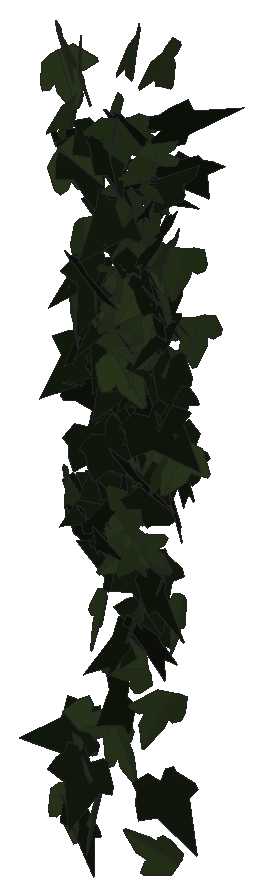
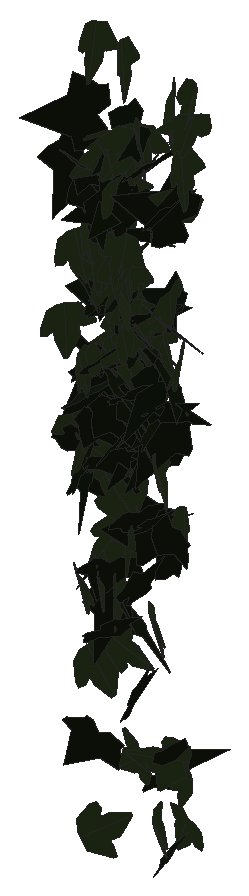
# SketchUp Ruby script. Lengths in inches.
U = 1.inch
M = Sketchup.active_model
def pt(a) = Geom::Point3d.new(a.map { |v| v * U })
def face(e, loops, mat)
  f = e.add_face(loops[0].map { |a| pt(a) })
  loops[1..].each { |l| e.add_face(l.map { |a| pt(a) }).erase! }
  f.material = f.back_material = mat if mat
  f
end
# faces: each face lists its corners as indices into pts; further lists are holes
def faces(e, pts, list, mat = nil) = list.each { |f| face(e, (f[0].is_a?(Array) ? f : [f]).map { |l| l.map { |i| pts[i] } }, mat) }
# xy, xz, yz: faces in a plane at the given z, y or x. An outline is a flat list of corners, or four numbers for a rectangle; further outlines are holes
def ring(l) = l.size == 4 ? [[l[0], l[1]], [l[2], l[1]], [l[2], l[3]], [l[0], l[3]]] : l.each_slice(2).to_a
def flat(e, list, mat, &to3) = list.each { |f| face(e, (f[0].is_a?(Array) ? f : [f]).map { |l| ring(l).map { |u, v| to3.(u, v) } }, mat) }
def xy(e, z, list, mat = nil) = flat(e, list, mat) { |x, y| [x, y, z] }
def xz(e, y, list, mat = nil) = flat(e, list, mat) { |x, z| [x, y, z] }
def yz(e, x, list, mat = nil) = flat(e, list, mat) { |y, z| [x, y, z] }
def lines(e, pts, list) = list.each { |a, b| e.add_line(pt(pts[a]), pt(pts[b])) }
# prism: a flat outline (further loops are holes) pulled along v
def prism(e, loops, v, mat = nil)
  f = face(e, loops, mat); d = Geom::Vector3d.new(v.map { |x| x * U })
  f.pushpull(f.normal.samedirection?(d) ? d.length : -d.length)
end
def box(e, o, s, mat = nil) = prism(e, [[o, [o[0] + s[0], o[1], o[2]], [o[0] + s[0], o[1] + s[1], o[2]], [o[0], o[1] + s[1], o[2]]]], [0, 0, s[2]], mat)
def at(x, y, z, deg = 0) = Geom::Transformation.translation(pt([x, y, z])) * Geom::Transformation.rotation(ORIGIN, Z_AXIS, deg.degrees)
def axes(o, x, y, z) = Geom::Transformation.new([*x, 0, *y, 0, *z, 0, *pt(o).to_a, 1])
def part(name) = M.definitions.add(name)
# library, detail: a bought-in or finely detailed component or shape, given as its bounding box
def library(name, o, s) = part(name).tap { |d| box(d.entities, o, s) }
def detail(e, o, s) = box(e.add_group.entities, o, s)
def put(e, d, t, mat = nil) = e.add_instance(d, t).tap { |i| i.material = mat if mat }
def group(e, t, mat = nil) = e.add_group.tap { |g| g.transformation = t; g.material = mat if mat }.entities
root = M.entities
M.materials.add("efeu1").color = [18, 25, 13]
M.materials.add("efeu2").color = [43, 57, 29]
c1 = part("ivyleaf_9")
p = [[1.54,2.16,1.25],[1.36,2.04,1.19],[-0.21,0.99,0.68],[-0.71,1.11,0.82],[-0.85,0.86,0.67],[-0.8,0.17,0.21],
  [-0.9,-0.01,0.1],[-0.67,-0.16,-0.02],[-0.08,-0.08,-0.05],[-0.03,-0.6,-0.4],[0.65,-0.88,-0.66],[0.83,-0.6,-0.49],
  [1.29,-0.42,-0.43],[1.8125,-0.07,-0.26],[1.21,0.44,0.15]]
faces(c1.entities,p,[[0,1,2,3,4,5,6,7,8,9,10,11,12,13,14]],"efeu1")
c2 = part("ivyleaf_10")
p = [[0,0.5,-0.03],[-0.0625,2.02,-0.43],[-0.19,2.01,-0.46],[-0.54,1.05,-0.29],[-0.52,0.625,-0.18],[-0.83,0.76,-0.28],
  [-1.16,0.64,-0.33],[-1.15,0.33,-0.24],[-0.77,-0.39,0.02],[-0.3,-0.51,0.16],[0.04,-0.48,0.23],[-0.02,2.01,-0.4375],
  [-0.06,2.01,-0.43],[0.04,-0.49,0.23],[0.67,-0.49,0.14],[1.38,0.36,-0.2],[1.375,0.51,-0.24],[0.81,0.65,-0.19],
  [0.62,0.59,-0.15],[0.6,1.09,-0.28],[0.5,1.23,-0.31]]
faces(c2.entities,p,[[0,1,2,3,4,5,6,7,8,9,10],[11,12,0,13,14,15,16,17,18,19,20]],"efeu2")
put(root,c1,axes([562.42,130.92,237.73],[0.53828,-0.80602,-0.202],[-0.09043,0.18243,-0.9689],[0.82601,0.54523,0.02556]))
put(root,c1,axes([563.375,131.01,223.55],[0.65129,-0.48232,0.57917],[0.49242,-0.30719,-0.80957],[0.5706,0.81562,0.03758]))
put(root,c1,axes([561.1875,131.4,209.32],[-0.31246,-0.89852,0.09086],[-0.02999,-0.08576,-0.9513],[0.9026,-0.3139,-0.00015]))
put(root,c1,axes([561.04,131.21,231.3],[0.42093,-0.46544,0.73818],[0.51312,-0.53091,-0.62735],[0.70587,0.66349,0.01585]))
put(root,c1,axes([561.99,131.15,238.16],[0.17865,-0.96038,-0.15125],[0.17379,0.18285,-0.95577],[0.95656,0.14614,0.20189]))
put(root,c2,axes([563.16,130.71,228.33],[0.71443,0.30335,0.61866],[0.54056,0.30587,-0.77422],[-0.42727,0.8942,0.05495]))
put(root,c2,axes([561.73,130.32,240.95],[-0.39643,0.28971,0.97126],[-0.77878,0.58041,-0.49098],[-0.64868,-0.87386,-0.00411]))
put(root,c2,axes([565.5,130.67,242.87],[-0.07993,-0.92921,-0.42172],[0.05156,0.41879,-0.93253],[1.01912,-0.09407,0.0141]))
put(root,c2,axes([564.62,130.75,236.61],[-0.9146,0.32449,0.01296],[-0.01122,0.00714,-0.97045],[-0.32456,-0.91466,-0.00298]))
put(root,c1,axes([565.01,130.58,226.54],[-0.14596,-0.31953,-0.94406],[0.31855,0.88913,-0.35019],[0.9444,-0.34929,-0.02778]))
put(root,c1,axes([564.41,130.8,232.36],[0.67031,-0.622,-0.34601],[-0.19163,0.30004,-0.91059],[0.68548,0.69211,0.08379]))
put(root,c1,axes([563.4,130.91,215.93],[-0.80632,0.58689,-0.0241],[0.01185,-0.02466,-0.99721],[-0.58727,-0.80631,0.01296]))
put(root,c2,axes([563.54,130.99,235.85],[-0.65715,0.56335,-0.47401],[0.37812,-0.28693,-0.86521],[-0.63172,-0.75776,-0.02478]))
put(root,c1,axes([565.68,131.09,231.25],[-0.96323,0.50519,-0.32722],[0.28967,-0.15219,-1.08767],[-0.52762,-1.00584,0.00022]))
put(root,c2,axes([563.14,130.9,238.87],[-0.82898,-0.58294,-0.0186],[0.01115,0.01647,-1.0134],[0.58313,-0.82902,-0.00706]))
put(root,c2,axes([565.11,131.35,213.51],[-0.37294,-0.87684,0.45217],[-0.1122,-0.44256,-0.95076],[0.98016,-0.38429,0.06321]))
put(root,c2,axes([560.35,130.8125,241.84],[-0.77246,0.62242,0.08901],[-0.0651,0.06107,-0.992],[-0.62537,-0.77517,-0.00668]))
put(root,c1,axes([560.81,131.17,220.22],[0.46178,0.1007,-0.92747],[0.91364,0.16047,0.47232],[0.18867,-1.02357,-0.0172]))
put(root,c1,axes([564.52,130.97,218.94],[0.67957,-0.63242,-0.33134],[-0.22317,0.24635,-0.92794],[0.67818,0.71478,0.02666]))
put(root,c1,axes([562.83,131.7,234.74],[-0.81509,-0.53147,0.11797],[0.04162,-0.27261,-0.94058],[0.54282,-0.77715,0.24926]))
put(root,c1,axes([563.21,130.78,239.23],[1.00852,-0.06202,-0.08568],[-0.08469,0.01875,-1.01034],[0.06338,1.01198,0.01347]))
put(root,c2,axes([563.74,131.01,242.74],[0.28145,-0.94142,-0.25988],[-0.00186,0.26994,-0.97987],[0.97663,0.27182,0.07303]))
put(root,c2,axes([562.89,131.58,232.83],[0.26327,-0.71145,0.6138],[0.45024,-0.46398,-0.73091],[0.82474,0.4804,0.20308]))
put(root,c2,axes([563.62,131.4,236.32],[-0.34525,-0.90146,0.24674],[-0.02997,-0.25222,-0.96343],[0.93414,-0.34126,0.06028]))
put(root,c2,axes([564.58,131.3,231.3],[0.94867,-0.22191,0.05992],[0.05955,-0.0085,-0.97426],[0.22201,0.95052,0.00527]))
put(root,c2,axes([563.8125,131.36,231.99],[0.8586,0.38619,-0.3853],[-0.36742,-0.1217,-0.94074],[-0.40324,0.93319,0.03677]))
put(root,c2,axes([562.69,131.36,239.25],[0.6154,-0.78959,0.04184],[0.09138,0.01836,-0.99762],[0.7854,0.61654,0.08328]))
put(root,c2,axes([564.27,131.65,228.75],[-0.36525,-0.76946,0.49291],[-0.0791,-0.50221,-0.84259],[0.91037,-0.35235,0.12455]))
put(root,c1,axes([564.98,131.26,209.82],[-0.30449,-0.36779,-0.9293],[0.73072,0.58084,-0.46931],[0.68185,-0.78672,0.08795]))
put(root,c2,axes([560.42,131.22,238.71],[0.06764,-0.98974,-0.17322],[-0.00006,0.17361,-0.99198],[1.00478,0.06664,0.01161]))
put(root,c1,axes([565.03,130.86,231.29],[0.0181,0.13265,-1.05903],[-1.0673,0.00589,-0.01751],[0.00367,1.05917,0.13273]))
put(root,c2,axes([560.14,131.03,240.64],[0.42511,0.86432,0.23318],[0.08388,0.21854,-0.96299],[-0.89128,0.43282,0.02059]))
put(root,c1,axes([562.86,131.15,229.47],[0.86,-0.39274,-0.06197],[-0.0508,0.03793,-0.94534],[0.39434,0.86139,0.01337]))
put(root,c2,axes([564.41,131.39,237.95],[0.66411,-0.72675,0.02418],[0.05594,0.01841,-0.98301],[0.72499,0.66429,0.0537]))
put(root,c2,axes([563.24,131.125,230.125],[-0.83326,-0.3656,-0.27601],[0.25782,0.09928,-0.90986],[0.37865,-0.87215,0.01213]))
put(root,c2,axes([563.79,131.36,214.59],[-0.26955,0.05015,0.89638],[-0.87007,-0.24532,-0.24792],[0.22133,-0.90331,0.11709]))
put(root,c1,axes([564.31,131.5,231.5],[0.61368,-0.6177,0.43655],[0.38239,-0.23167,-0.86535],[0.65261,0.71659,0.09654]))
put(root,c1,axes([565.86,131.27,237.02],[-0.70405,0.61197,0.32245],[-0.46019,-0.07089,-0.87026],[-0.51643,-0.77112,0.3359]))
put(root,c1,axes([564.25,130.97,216.58],[0.90189,0.14899,-0.53833],[-0.53266,-0.07835,-0.91408],[-0.16814,1.04741,0.0082]))
put(root,c2,axes([562.85,131.3,220.68],[0.57368,-0.03964,0.78885],[0.78367,0.15028,-0.56236],[-0.09861,0.96374,0.12013]))
put(root,c1,axes([562.49,132.1,212.51],[-0.07871,-0.49549,0.82496],[-0.1517,-0.81097,-0.50157],[0.95029,-0.1705,-0.01174]))
put(root,c2,axes([563.39,131.41,229.0625],[-0.74927,-0.55932,0.22375],[-0.15598,-0.16479,-0.93425],[0.58187,-0.7644,0.03769]))
put(root,c2,axes([560.67,130.82,236.61],[0.32302,0.79126,0.65933],[0.26155,0.60533,-0.85459],[-0.99619,0.4155,-0.01057]))
put(root,c1,axes([562.15,131.65,229.22],[-0.78545,-0.26057,-0.4574],[0.44405,0.11328,-0.82706],[0.28271,-0.90184,0.02827]))
put(root,c2,axes([563.29,131.78,219.8],[0.34467,0.38691,-0.74989],[-0.52499,-0.53585,-0.51777],[-0.66062,0.6277,0.02022]))
put(root,c1,axes([564.94,131.21,234.32],[-0.61236,0.77049,-0.02027],[0.01176,-0.01655,-0.98419],[-0.77067,-0.61247,0.00109]))
put(root,c1,axes([561.51,131.1,224.63],[0.19387,-0.58216,-0.75185],[-0.0458,0.76071,-0.60083],[0.94979,0.15551,0.1245]))
put(root,c2,axes([560.01,131.63,209.56],[-0.2914,0.19597,-0.84689],[0.69816,-0.47938,-0.35115],[-0.51788,-0.75653,0.00313]))
put(root,c1,axes([562.41,131.02,224.625],[0.21339,-0.50269,-0.82813],[-0.13631,0.82397,-0.53529],[0.95913,0.22894,0.10818]))
put(root,c1,axes([561.76,132.11,221.22],[-0.58473,-0.44155,0.53269],[-0.20908,-0.55207,-0.68712],[0.65955,-0.56647,0.25443]))
put(root,c2,axes([565.2,131.48,233.97],[0.1906,-0.96153,-0.07796],[-0.04752,0.07002,-0.97969],[0.96352,0.19366,-0.03289]))
put(root,c2,axes([561.61,131.65,216.6],[0.70348,-0.63415,0.16529],[0.12314,-0.11025,-0.94712],[0.64366,0.71418,0.00055]))
put(root,c2,axes([564.49,130.98,237.91],[-0.42808,-0.40328,-0.79271],[0.578,0.5425,-0.58812],[0.67597,-0.71926,0.00088]))
put(root,c1,axes([561.53,132,231.39],[-0.51304,-0.81769,0.05598],[-0.00209,-0.06474,-0.96476],[0.8196,-0.51201,0.03259]))
put(root,c2,axes([560.45,131.24,221.6875],[-0.69677,0.43299,0.38568],[-0.39566,0.08574,-0.81106],[-0.42389,-0.79177,0.12309]))
put(root,c1,axes([565.01,131.74,228.62],[-0.72665,-0.26809,-0.54356],[0.52634,0.14162,-0.77348],[0.3005,-0.89634,0.04037]))
put(root,c2,axes([559.84,131.59,207.44],[0.77248,-0.15436,0.51226],[0.51575,-0.02442,-0.78509],[0.14228,0.92657,0.06465]))
put(root,c1,axes([560.67,131.63,236.63],[0.18606,-0.92804,-0.29168],[-0.00811,0.29547,-0.9453],[0.97277,0.17997,0.04791]))
put(root,c1,axes([563.91,131.35,221.91],[-0.35705,0.16504,0.90378],[0.82784,-0.36269,0.39329],[0.39841,0.90153,-0.00723]))
put(root,c1,axes([560.6,132.07,210.22],[-0.43311,-0.21345,0.80804],[-0.68721,-0.42699,-0.48113],[0.47563,-0.81129,0.04063]))
put(root,c2,axes([563.3,131.1875,238.68],[-0.70156,-0.464,-0.53052],[0.43122,0.3095,-0.84095],[0.55749,-0.82332,-0.01715]))
put(root,c1,axes([562.24,131.93,230.26],[-0.89135,0.05033,-0.37053],[0.34062,-0.2859,-0.85823],[-0.15428,-0.92198,0.24591]))
put(root,c1,axes([563.01,131.48,232.06],[0.89354,-0.43294,0.04999],[0.04215,-0.02765,-0.99288],[0.43377,0.89451,-0.00649]))
put(root,c1,axes([563.52,130.84,236.1875],[0.72775,0.63648,0.2004],[-0.00938,0.30626,-0.93863],[-0.66722,0.68992,0.23178]))
put(root,c2,axes([565.68,131.69,224.75],[0.76153,0.42114,-0.32079],[-0.29083,-0.1368,-0.87],[-0.44237,0.81494,0.01974]))
put(root,c2,axes([563.28,131.48,221.48],[-0.67994,-0.4683,0.53221],[0.43598,0.30527,0.8256],[-0.55901,0.8077,-0.00346]))
put(root,c2,axes([561.69,131.2,229.93],[-0.34573,0.15548,0.96307],[-0.90678,0.32558,-0.37808],[-0.35975,-0.97007,0.02747]))
put(root,c2,axes([562.57,132.12,230.12],[-0.11019,-0.75305,0.59379],[0.16482,-0.60367,-0.735],[0.94472,0.01749,0.19748]))
put(root,c2,axes([563.83,131.22,219.95],[-0.4883,-0.5347,-0.62054],[0.41005,0.46583,-0.72406],[0.7091,-0.63758,-0.00862]))
put(root,c2,axes([563.62,131.58,231.66],[-0.89285,-0.33818,0.05586],[-0.03147,-0.07432,-0.95297],[0.34132,-0.89151,0.05826]))
put(root,c1,axes([562.48,132.29,227.3125],[-0.52994,-0.75342,0.2715],[-0.00488,-0.32251,-0.90452],[0.80083,-0.50054,0.17415]))
put(root,c2,axes([561.8,131.53,230.5],[0.79029,0.54311,0.12149],[0.04134,0.15313,-0.95348],[-0.555,0.78477,0.10197]))
put(root,c2,axes([563.84,131.24,217.49],[0.22607,-0.76514,-0.70773],[-0.19305,0.68091,-0.79781],[1.02423,0.29723,0.00584]))
put(root,c2,axes([565.6,131.84,233.44],[-0.52327,-0.80541,0.20904],[-0.03132,-0.2277,-0.9557],[0.83151,-0.51542,0.09555]))
put(root,c1,axes([562.83,131.41,233.39],[0.69053,-0.57375,-0.43415],[-0.14086,0.4823,-0.86143],[0.70557,0.65781,0.25292]))
put(root,c1,axes([560.54,131.85,221.4375],[-0.36142,-0.14762,-0.92172],[0.87096,0.30226,-0.38992],[0.33583,-0.94277,0.01931]))
put(root,c1,axes([564.17,132.2,228.28],[-0.07847,-0.95567,0.04922],[0.09585,-0.05699,-0.95365],[0.95213,-0.07302,0.10006]))
put(root,c1,axes([565,131.37,236.17],[-0.10752,0.97207,-0.1177],[0.01891,-0.11632,-0.97798],[-0.97898,-0.109,-0.00596]))
put(root,c1,axes([561.95,131.05,220.25],[0.2654,0.09517,0.92197],[0.68316,0.62804,-0.26148],[-0.6264,0.72527,0.10545]))
put(root,c2,axes([560.96,132.19,207.11],[0.50971,-0.55797,0.59763],[0.3885,-0.45439,-0.75557],[0.71941,0.6407,-0.0154]))
put(root,c1,axes([560.67,132.34,227.17],[-0.73203,-0.49642,0.31362],[-0.19582,-0.26614,-0.87834],[0.55357,-0.75059,0.10402]))
put(root,c2,axes([564.45,131.97,223.77],[-0.31048,-0.06045,0.86319],[-0.76179,-0.41586,-0.30313],[0.4104,-0.81765,0.09036]))
put(root,c2,axes([563.13,131.76,233.02],[-0.92174,-0.29114,0.09967],[-0.07245,-0.10058,-0.96381],[0.29908,-0.92164,0.0737]))
put(root,c1,axes([563.55,131.57,227.33],[-0.59086,0.70866,0.1372],[-0.1198,0.07857,-0.92175],[-0.71181,-0.60147,0.04125]))
put(root,c1,axes([560.24,131.65,236.27],[0.52909,-0.12814,0.96083],[0.93442,-0.22372,-0.54439],[0.25781,1.07382,0.00124]))
put(root,c1,axes([562.78,131.4375,226.38],[-0.33671,0.86964,0.09789],[-0.10352,0.06457,-0.9297],[-0.86899,-0.34466,0.07282]))
put(root,c1,axes([562.37,132.27,225.72],[0.2939,-0.86361,0.2712],[0.06008,-0.2659,-0.91183],[0.90319,0.29871,-0.0276]))
put(root,c1,axes([560.05,132.23,206.41],[0.34625,-0.84368,0.2148],[0.07241,-0.20245,-0.91192],[0.86758,0.35361,-0.00962]))
put(root,c2,axes([560.03,131.91,229.71],[-0.37643,0.86082,-0.25507],[0.06112,-0.25136,-0.93854],[-0.89573,-0.37891,0.04314]))
put(root,c2,axes([562.53,132.28,231.87],[0.28244,-0.82574,0.40425],[0.11507,-0.38782,-0.87257],[0.91215,0.30461,-0.01509]))
put(root,c1,axes([561.03,132.24,231.61],[-0.94168,0.09839,-0.16926],[0.14342,-0.21934,-0.92542],[-0.13327,-0.93129,0.20007]))
put(root,c2,axes([565.09,131.37,224.35],[-0.08601,-0.67643,-0.77219],[0.10937,0.76444,-0.68183],[1.02072,-0.13891,0.00799]))
put(root,c2,axes([565.15,132.12,217.48],[0.74448,-0.49476,0.19832],[0.16368,-0.11202,-0.89388],[0.50727,0.76225,-0.00264]))
put(root,c1,axes([563.18,131.51,235.95],[0.79679,0.12443,0.54979],[0.5443,0.07771,-0.80642],[-0.14658,0.96493,-0.00595]))
put(root,c2,axes([564.08,131.85,233.42],[-0.95473,0.1922,0.0086],[-0.02603,-0.08591,-0.96978],[-0.19062,-0.9509,0.08935]))
put(root,c1,axes([565.17,131.1875,239.33],[0.55237,0.18946,0.9452],[0.77509,0.56045,-0.5653],[-0.57319,0.94044,0.14646]))
put(root,c1,axes([565.21,131.52,222.64],[0.47719,-0.06255,-0.84979],[-0.82037,0.22953,-0.47757],[0.23031,0.94719,0.05961]))
put(root,c1,axes([562.84,131.42,230.19],[-0.14957,0.48576,0.81588],[-0.47068,0.67939,-0.49079],[-0.82467,-0.47587,0.13214]))
put(root,c1,axes([560.97,131.46,226.15],[0.83396,0.60909,-0.12871],[-0.10362,-0.07635,-1.0327],[-0.61385,0.84037,-0.00053]))
put(root,c1,axes([562.1,132.52,218.04],[-0.24729,0.19387,0.87259],[-0.5971,-0.70956,-0.01157],[0.66518,-0.56487,0.31401]))
put(root,c1,axes([563.52,132.19,218.83],[-0.2655,-0.78685,-0.50479],[0.2433,0.44851,-0.82709],[0.90264,-0.35234,0.07446]))
put(root,c2,axes([560.4,132.14,232.7],[-0.02512,0.92926,-0.26709],[-0.01269,-0.26748,-0.9294],[-0.9668,-0.02063,0.01914]))
put(root,c1,axes([560.85,131.36,228.19],[-0.19799,0.67605,0.75201],[-0.21286,0.72125,-0.70444],[-0.98856,-0.2907,0.00107]))
put(root,c1,axes([561.12,132.1,226.55],[0.72227,-0.61928,-0.08191],[-0.06734,0.0473,-0.95138],[0.62104,0.72536,-0.00789]))
put(root,c2,axes([564.34,132.02,218.57],[0.45841,-0.82523,-0.32812],[-0.13783,0.29867,-0.94372],[0.87731,0.47812,0.02318]))
put(root,c2,axes([562.16,132.02,231.3125],[-0.94263,-0.21997,-0.04757],[0.04844,0.00174,-0.96791],[0.21978,-0.94382,0.0093]))
put(root,c2,axes([562.98,131.99,234.2],[-0.97037,0.08047,0.01787],[-0.01793,0.00006,-0.9737],[-0.08046,-0.97053,0.00142]))
put(root,c1,axes([561.73,132.45,221.97],[-0.17034,-0.89138,-0.29933],[0.12422,0.28021,-0.90511],[0.93205,-0.20025,0.06592]))
put(root,c1,axes([565.42,132.58,224.47],[-0.8428,-0.26458,0.25581],[-0.24914,-0.06034,-0.88321],[0.27088,-0.8787,-0.01638]))
put(root,c2,axes([564.34,132.39,205.8],[-0.51174,0.01002,-0.83275],[-0.82443,-0.14439,0.50489],[-0.11784,0.9667,0.08404]))
put(root,c1,axes([565.46,131.68,237.48],[0.64612,0.74725,-0.03278],[-0.0166,-0.02899,-0.98783],[-0.74778,0.6463,-0.0064]))
put(root,c1,axes([564.21,132.73,226.96],[-0.02243,-0.89944,0.19745],[0.30443,-0.19365,-0.84753],[0.86908,0.04462,0.30197]))
put(root,c1,axes([563.14,132.37,226.81],[-0.08825,0.67183,-0.67181],[0.03693,-0.67176,-0.67664],[-0.94938,-0.08858,0.03613]))
put(root,c1,axes([561.22,131.98,228.18],[0.9314,-0.09802,-0.35514],[-0.3523,0.04552,-0.93651],[0.10779,0.99577,0.00785]))
put(root,c1,axes([563.33,132.95,216.1],[-0.52173,-0.73579,0.27179],[-0.02677,-0.30953,-0.88934],[0.78392,-0.50026,0.15052]))
put(root,c2,axes([561.75,132.49,210.3],[0.5721,-0.09006,0.82312],[0.81315,-0.12771,-0.57915],[0.15627,0.99424,0.00016]))
put(root,c2,axes([560.79,132.4,224.57],[0.42124,-0.84181,-0.02418],[-0.00648,0.02379,-0.94131],[0.84214,0.42126,0.00485]))
put(root,c2,axes([564.71,132.59,228.21],[0.26727,-0.84253,0.30621],[0.25057,-0.23658,-0.86965],[0.86071,0.33049,0.15809]))
put(root,c2,axes([562.64,132.11,220.68],[0.64443,-0.57343,-0.28787],[-0.01595,0.39356,-0.81966],[0.64143,0.5859,0.26884]))
put(root,c1,axes([562.68,132.8,225.21],[0.12536,-0.87706,0.22262],[0.02256,-0.22165,-0.88593],[0.90459,0.12707,-0.00875]))
put(root,c1,axes([563.23,132.81,224.32],[-0.5357,-0.73522,-0.04467],[0.07152,0.00305,-0.90797],[0.7331,-0.53755,0.05594]))
put(root,c2,axes([560.22,131.85,210.43],[0.14735,0.12175,-1.01603],[0.87748,0.51309,0.18874],[0.52647,-0.88925,-0.03021]))
put(root,c1,axes([563.78,132.7,226.3],[-0.15649,0.49308,-0.76149],[0.14489,-0.74923,-0.51492],[-0.89555,-0.20738,0.04976]))
put(root,c1,axes([564.48,133,223.12],[0.18754,-0.58114,0.69296],[0.18305,-0.66866,-0.61031],[0.88567,0.26125,-0.0206]))
put(root,c2,axes([565.71,132.5,230.14],[-0.56093,-0.76683,0.04934],[0.06511,-0.1083,-0.94294],[0.76565,-0.55259,0.11633]))
